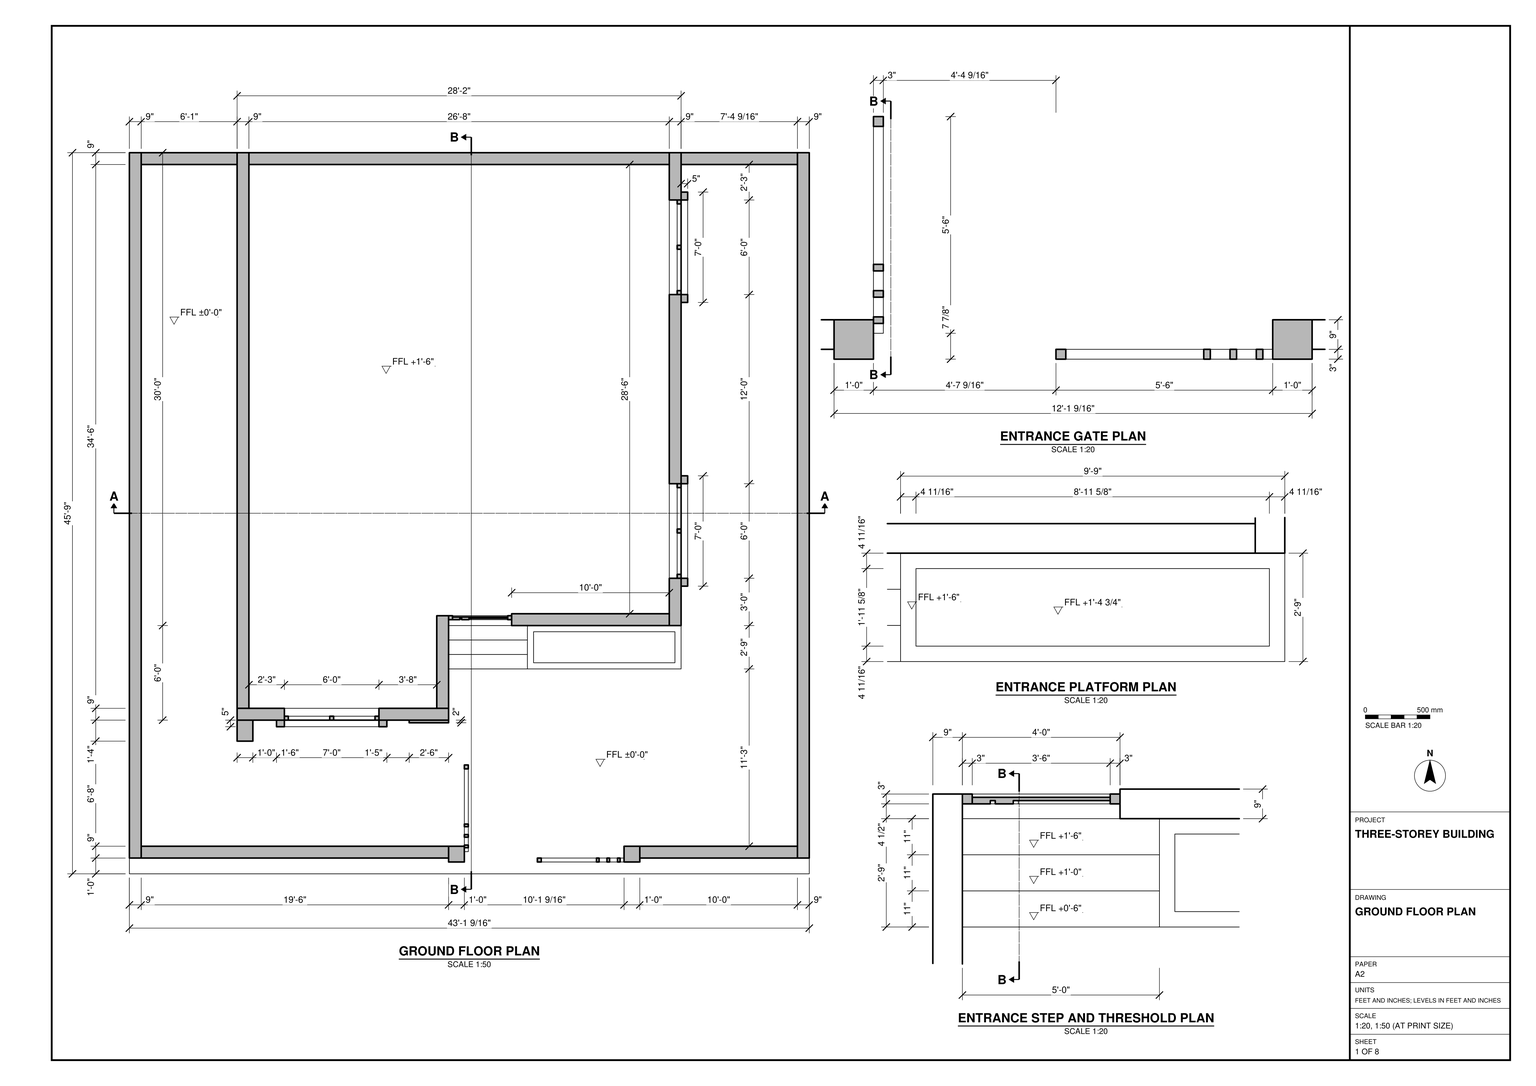
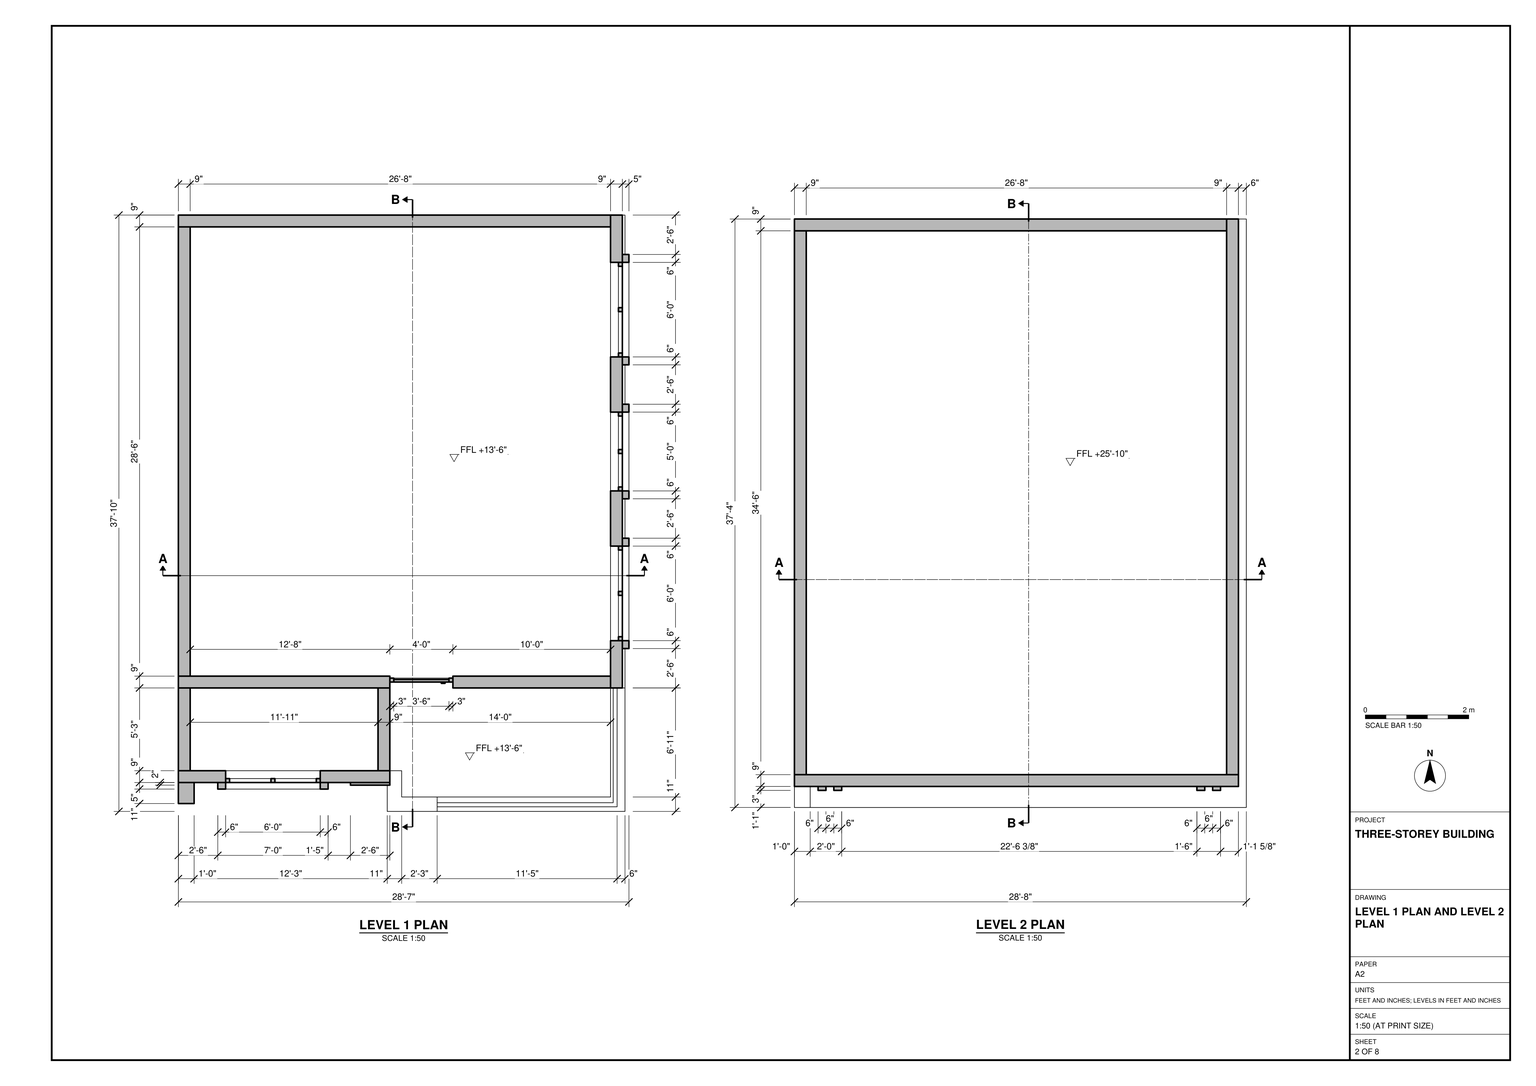
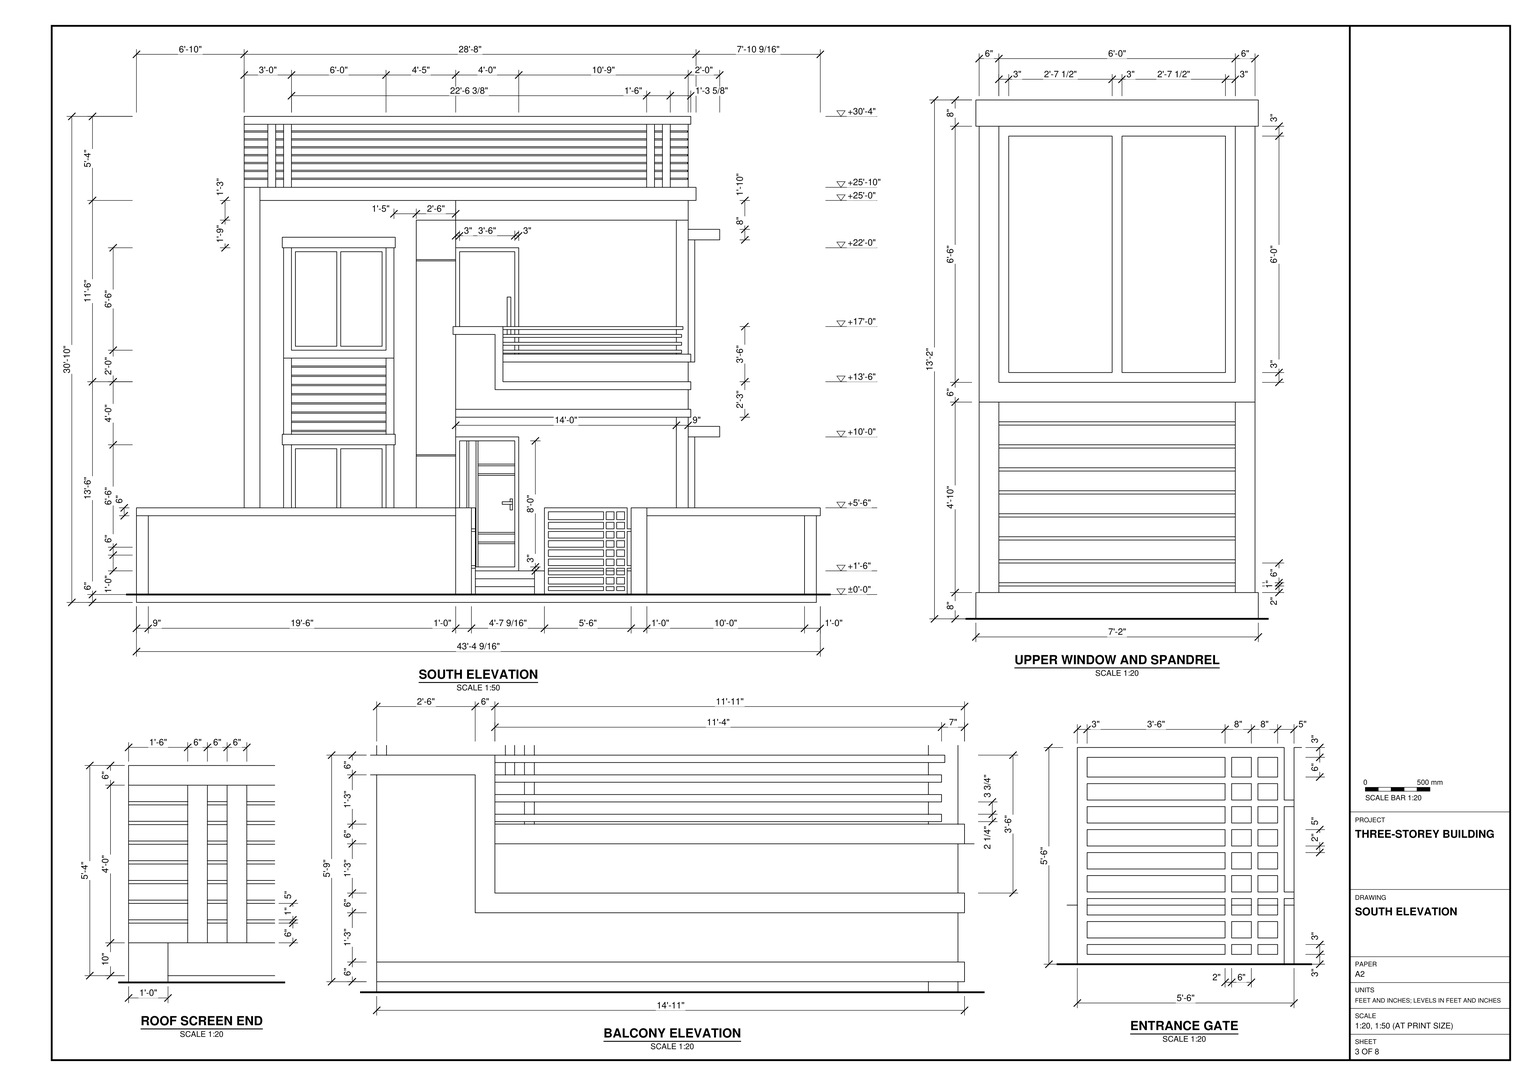
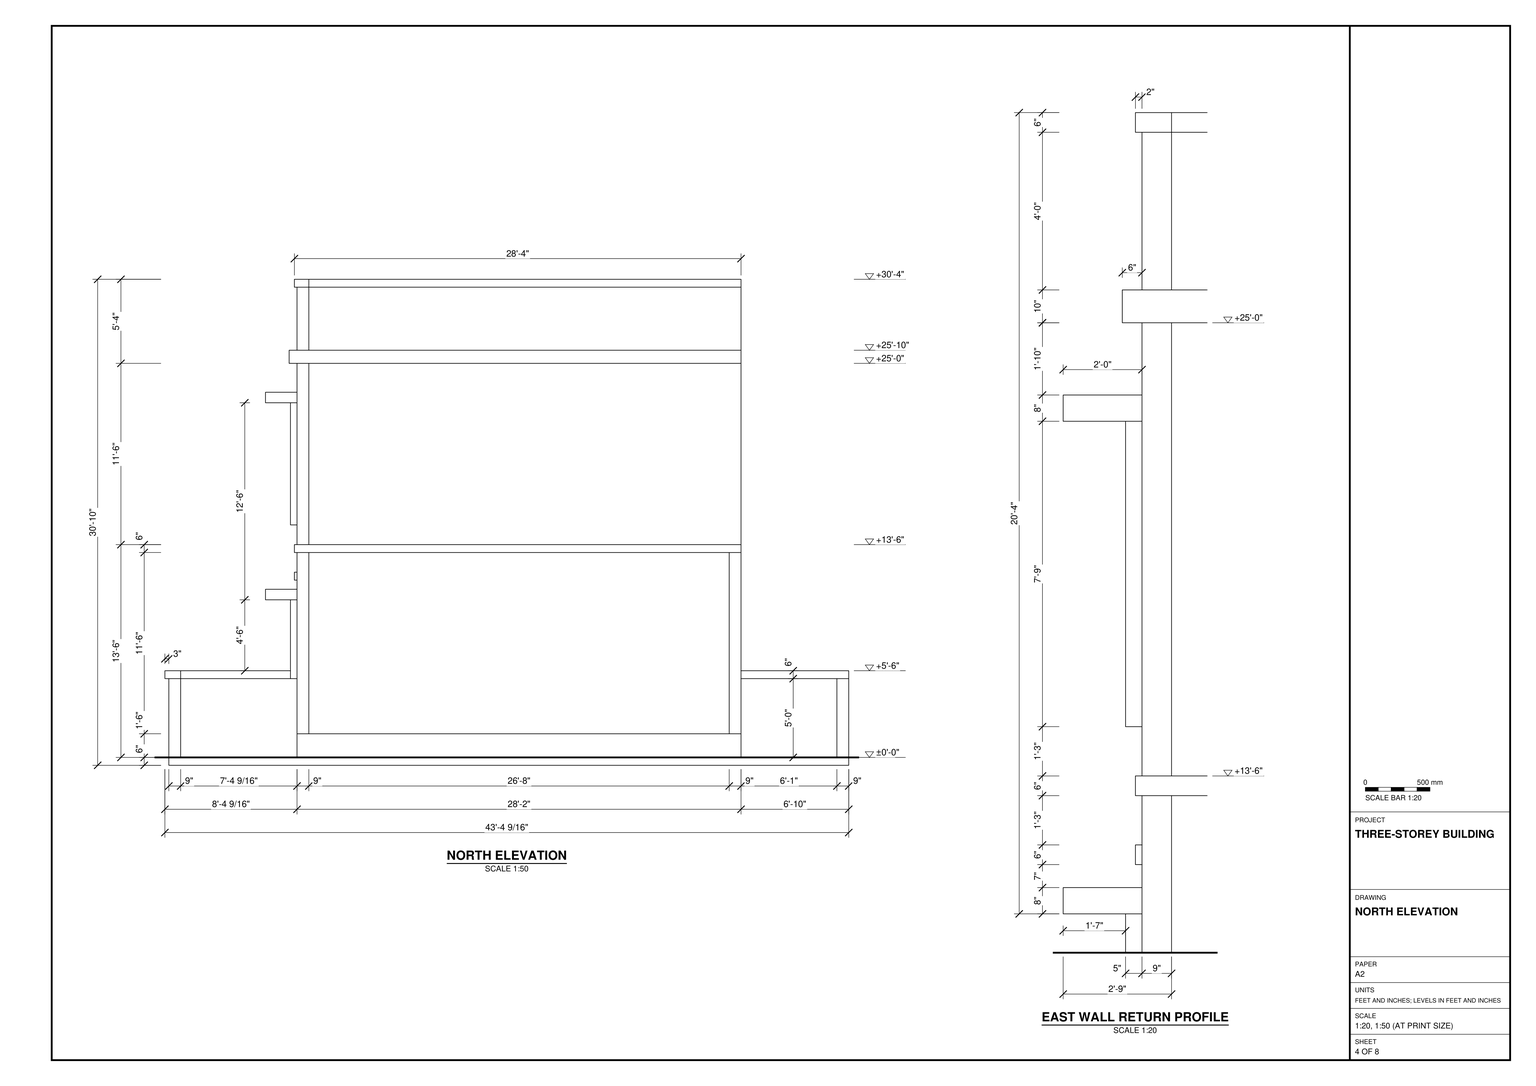
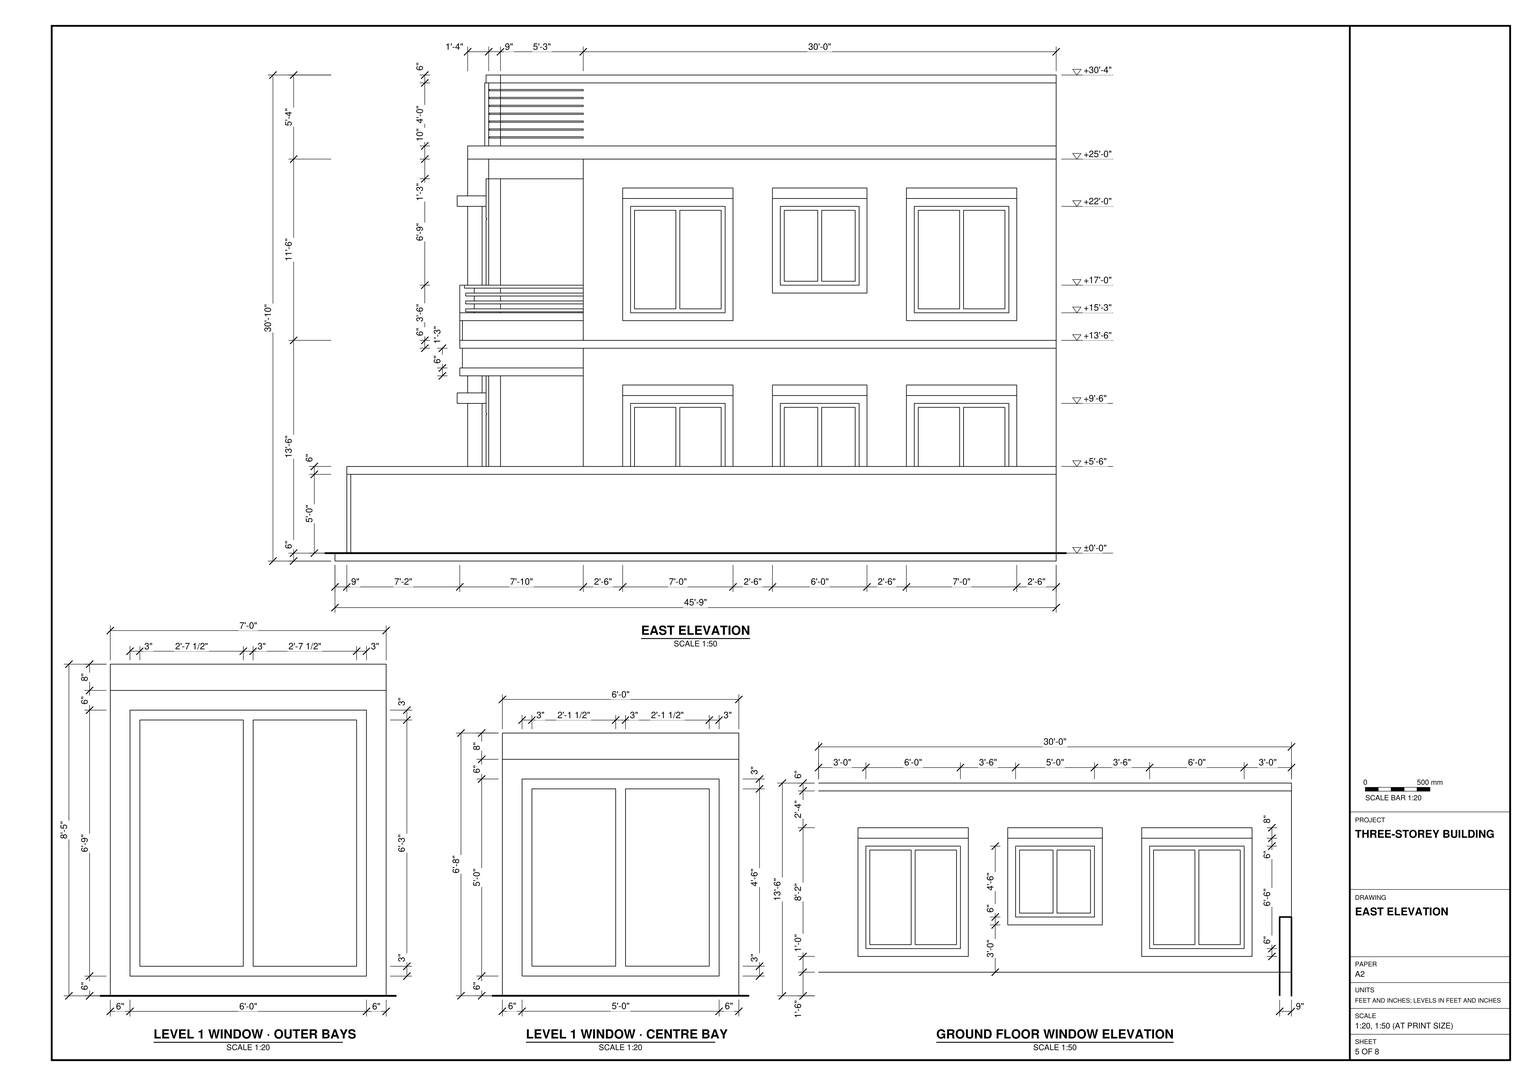
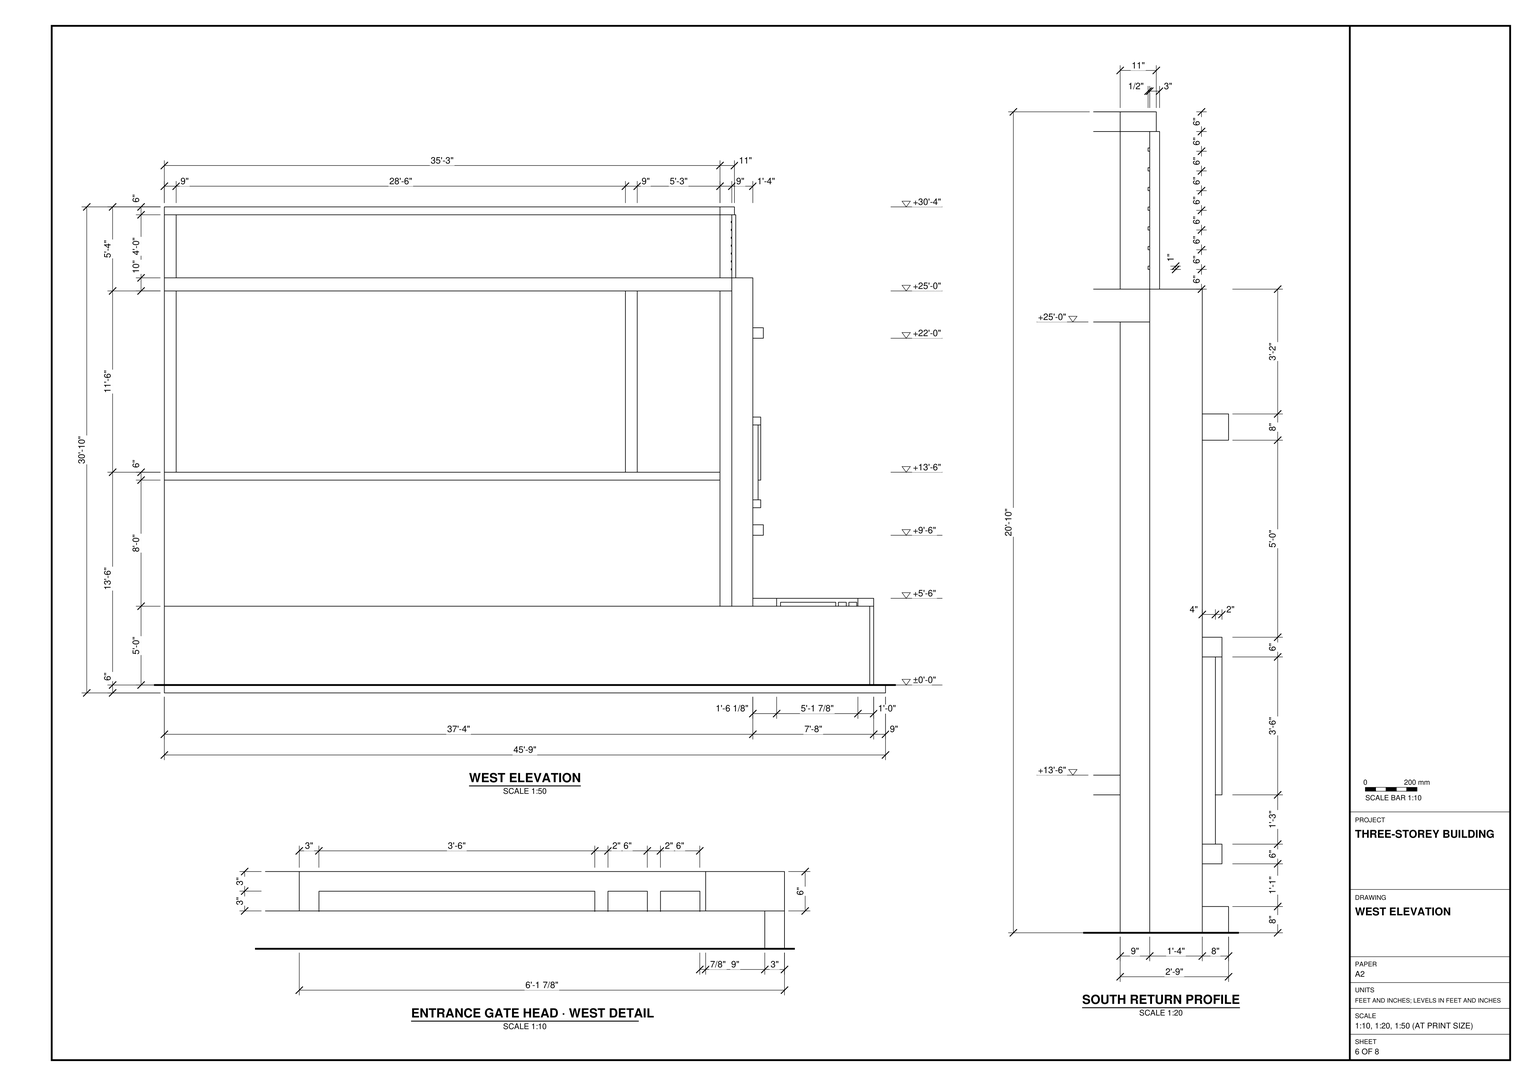
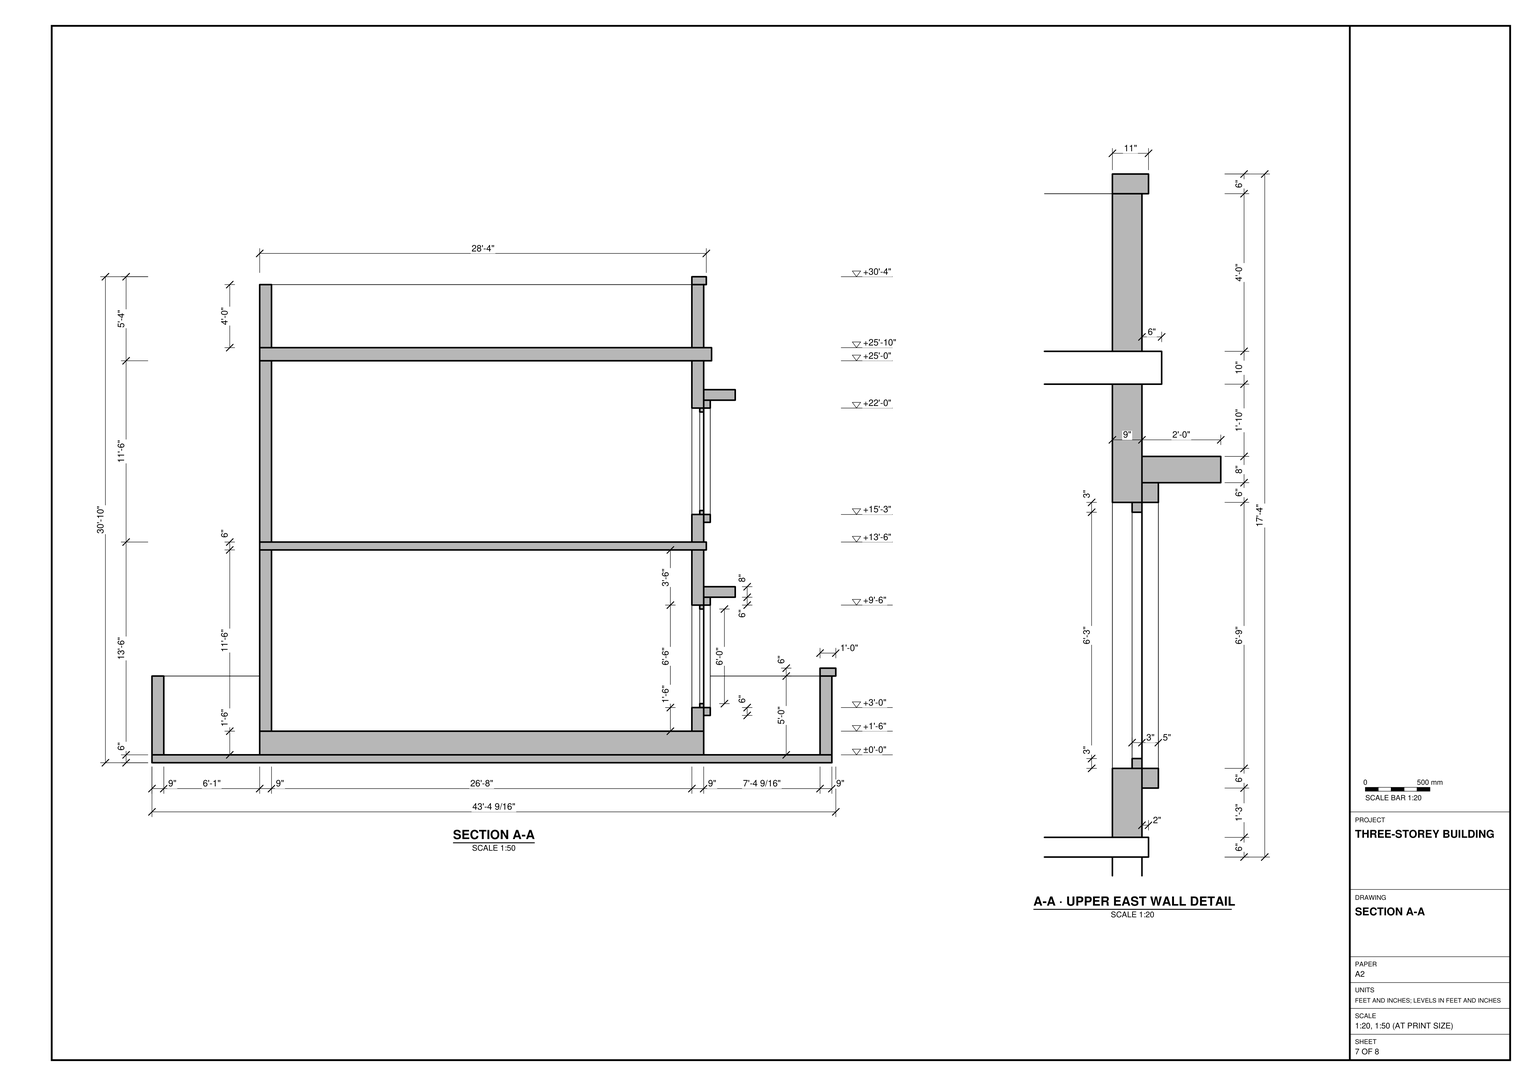
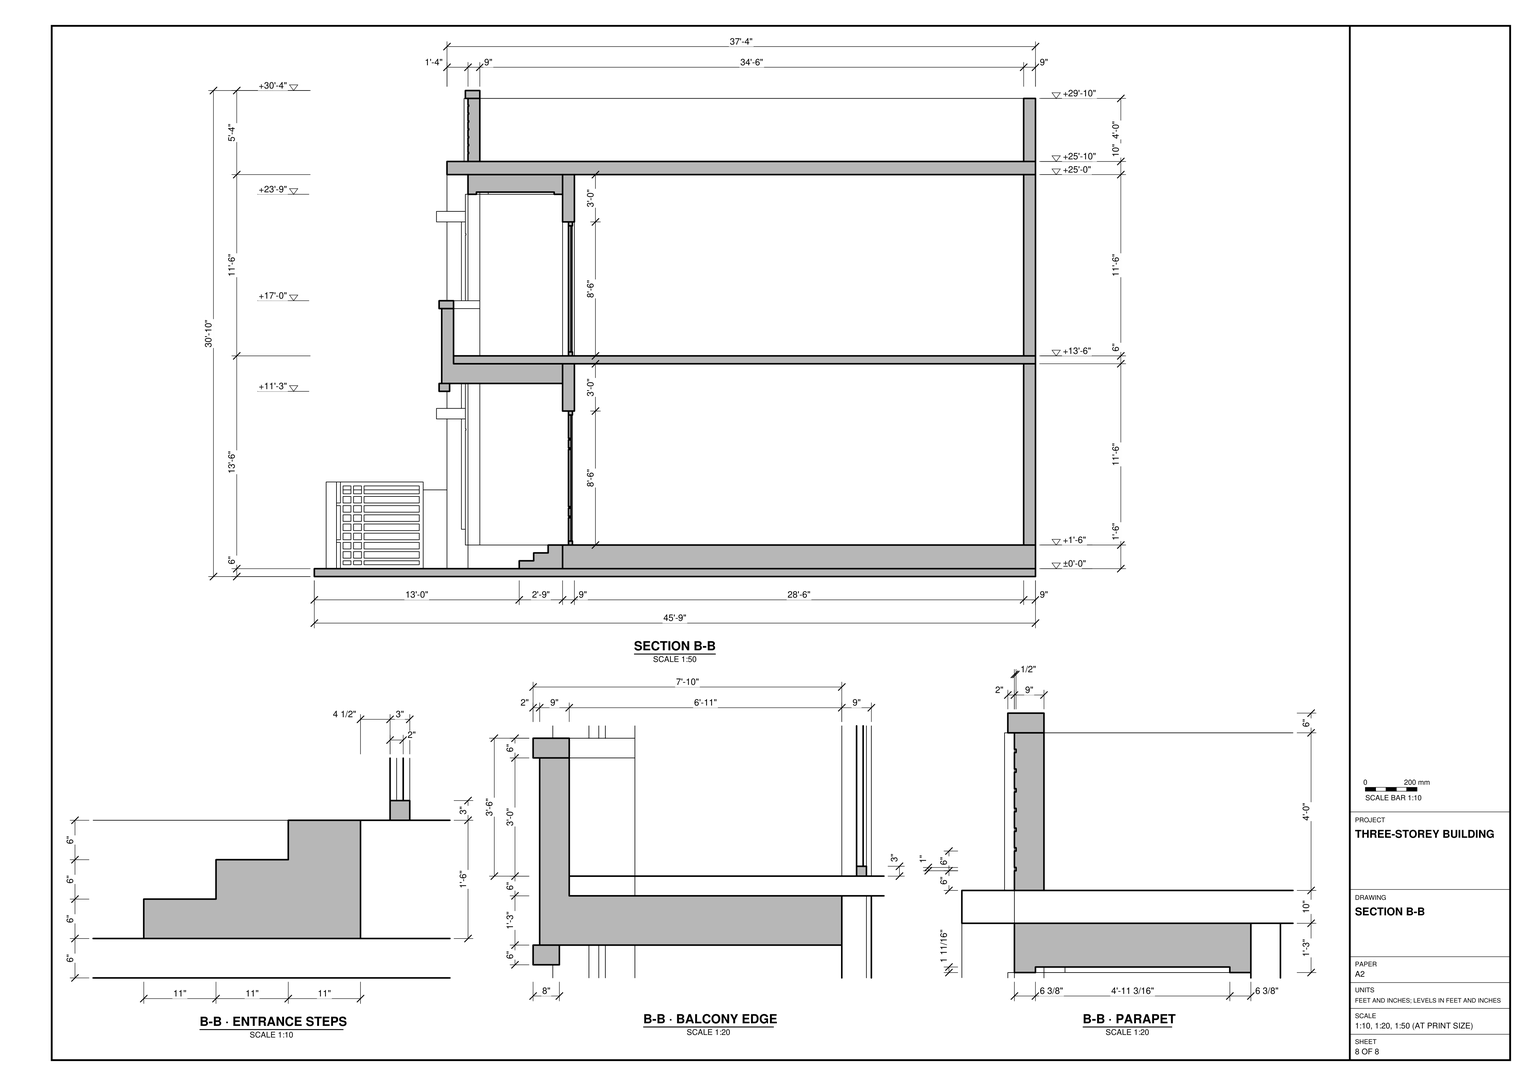
Build the three-storey building and its walled forecourt in SketchUp using task_files/diagram_01.pdf. Work in feet and inches. The overall model is 43'-4 9/16" across the south frontage, 45'-9" from front to back and 30'-10" from its lowest to its highest point. Use ±0'-0", +13'-6" and +25'-0" as the level references. Distinguish the forecourt at ±0'-0" from the raised ground-floor interior at +1'-6".

Lay out the boundary walls, gateposts and gate leaves from the ground-floor plan. Set the building back from the gate, with the projecting window bay to the left of the recessed entrance. Model the entrance steps, threshold and adjoining platform. Give the walls their drawn thicknesses, including the 9" main walls, and cut the door and window openings through them. Align the south windows vertically with the slatted spandrel between them. On the upper floor, model the door onto the front balcony, its solid lower face and its horizontal rails. Follow the plans for the east windows, floor slabs and flat roof, and use the elevation detail for the slats, uprights and cap of the roof screen.

Keep walls, slabs, roof elements and any furniture or joinery pieces in separate groups or components; use components for repeated parts. Decor and loose items, if included, may be any suitable library components. Save one SketchUp model as output_files/three_storey_building_with_gated_forecourt_and_balcony.skp.

# SketchUp Ruby script. Lengths in inches.
U = 1.inch
M = Sketchup.active_model
def pt(a) = Geom::Point3d.new(a.map { |v| v * U })
def face(e, loops, mat)
  f = e.add_face(loops[0].map { |a| pt(a) })
  loops[1..].each { |l| e.add_face(l.map { |a| pt(a) }).erase! }
  f.material = f.back_material = mat if mat
  f
end
# faces: each face lists its corners as indices into pts; further lists are holes
def faces(e, pts, list, mat = nil) = list.each { |f| face(e, (f[0].is_a?(Array) ? f : [f]).map { |l| l.map { |i| pts[i] } }, mat) }
# xy, xz, yz: faces in a plane at the given z, y or x. An outline is a flat list of corners, or four numbers for a rectangle; further outlines are holes
def ring(l) = l.size == 4 ? [[l[0], l[1]], [l[2], l[1]], [l[2], l[3]], [l[0], l[3]]] : l.each_slice(2).to_a
def flat(e, list, mat, &to3) = list.each { |f| face(e, (f[0].is_a?(Array) ? f : [f]).map { |l| ring(l).map { |u, v| to3.(u, v) } }, mat) }
def xy(e, z, list, mat = nil) = flat(e, list, mat) { |x, y| [x, y, z] }
def xz(e, y, list, mat = nil) = flat(e, list, mat) { |x, z| [x, y, z] }
def yz(e, x, list, mat = nil) = flat(e, list, mat) { |y, z| [x, y, z] }
def lines(e, pts, list) = list.each { |a, b| e.add_line(pt(pts[a]), pt(pts[b])) }
# prism: a flat outline (further loops are holes) pulled along v
def prism(e, loops, v, mat = nil)
  f = face(e, loops, mat); d = Geom::Vector3d.new(v.map { |x| x * U })
  f.pushpull(f.normal.samedirection?(d) ? d.length : -d.length)
end
def box(e, o, s, mat = nil) = prism(e, [[o, [o[0] + s[0], o[1], o[2]], [o[0] + s[0], o[1] + s[1], o[2]], [o[0], o[1] + s[1], o[2]]]], [0, 0, s[2]], mat)
def at(x, y, z, deg = 0) = Geom::Transformation.translation(pt([x, y, z])) * Geom::Transformation.rotation(ORIGIN, Z_AXIS, deg.degrees)
def axes(o, x, y, z) = Geom::Transformation.new([*x, 0, *y, 0, *z, 0, *pt(o).to_a, 1])
def part(name) = M.definitions.add(name)
# library, detail: a bought-in or finely detailed component or shape, given as its bounding box
def library(name, o, s) = part(name).tap { |d| box(d.entities, o, s) }
def detail(e, o, s) = box(e.add_group.entities, o, s)
def put(e, d, t, mat = nil) = e.add_instance(d, t).tap { |i| i.material = mat if mat }
def group(e, t, mat = nil) = e.add_group.tap { |g| g.transformation = t; g.material = mat if mat }.entities
root = M.entities
M.materials.add("[Aluminum]").color = [179, 179, 179]
M.materials.add("[Color C01]").color = [247, 234, 234]
M.materials.add("[Color C02]").color = [183, 146, 110]
M.materials.add("[Color M00]").color = [255, 255, 255]
M.materials.add("[Color M02]").color = [198, 198, 198]
M.materials.add("[Color M06]").color = [86, 86, 86]
M.materials.add("[Color M07]").color = [58, 58, 58]
M.materials.add("[Grass Dark Green]").color = [106, 157, 55]
M.materials.add("[Translucent Glass Gray]").color = [128, 128, 128]
M.materials["[Translucent Glass Gray]"].alpha = 0.5
M.materials.add("[Wood Veneer 01]").color = [120, 70, 37]
c1 = part("Group\#74")
box(c1.entities,[0,0,0],[6,3,48])
box(c1.entities,[12,0,0],[6,3,48])
c2 = part("Group\#93")
prism(c2.entities,[[[0,0,0],[63,0,0],[63,0,20],[66,0,20],[66,0,22],[63,0,22],[63,0,48],[66,0,48],[66,0,50],[63,0,50],[63,0,66],[0,0,66]],[[3,0,63],[45,0,63],[45,0,57],[3,0,57]],[[3,0,13],[45,0,13],[45,0,8],[3,0,8]],[[3,0,20],[45,0,20],[45,0,15],[3,0,15]],[[3,0,27],[45,0,27],[45,0,22],[3,0,22]],[[3,0,34],[45,0,34],[45,0,29],[3,0,29]],[[3,0,41],[45,0,41],[45,0,36],[3,0,36]],[[3,0,48],[45,0,48],[45,0,43],[3,0,43]],[[45,0,55],[45,0,50],[3,0,50],[3,0,55]],[[45,0,6],[45,0,3],[3,0,3],[3,0,6]],[[55,0,63],[61,0,63],[61,0,57],[55,0,57]],[[53,0,57],[47,0,57],[47,0,63],[53,0,63]],[[61,0,8],[55,0,8],[55,0,13],[61,0,13]],[[61,0,20],[61,0,15],[55,0,15],[55,0,20]],[[53,0,15],[47,0,15],[47,0,20],[53,0,20]],[[61,0,27],[61,0,22],[55,0,22],[55,0,27]],[[53,0,29],[47,0,29],[47,0,34],[53,0,34]],[[53,0,41],[53,0,36],[47,0,36],[47,0,41]],[[53,0,48],[53,0,43],[47,0,43],[47,0,48]],[[61,0,50],[55,0,50],[55,0,55],[61,0,55]],[[53,0,50],[47,0,50],[47,0,55],[53,0,55]],[[61,0,48],[61,0,43],[55,0,43],[55,0,48]],[[61,0,41],[61,0,36],[55,0,36],[55,0,41]],[[61,0,29],[55,0,29],[55,0,34],[61,0,34]],[[53,0,27],[53,0,22],[47,0,22],[47,0,27]],[[53,0,8],[47,0,8],[47,0,13],[53,0,13]],[[61,0,6],[61,0,3],[55,0,3],[55,0,6]],[[47,0,3],[47,0,6],[53,0,6],[53,0,3]]],[0,3,0])
p = [[66,3,22],[66,3,48],[66,3,0],[66,3,20],[66,3,50],[66,3,66]]
lines(c2.entities,p,[[0,1],[2,3],[4,5]])
p = [[94,112.99,306],[94,116.99,306]]
lines(root,p,[[0,1]])
g1 = group(root,at(142.63,241.1875,0))
box(g1,[-142.63,-241.1875,0],[517.57,548.99,6])
g2 = group(root,at(180,308.99,6),"[Color C01]")
prism(g2,[[[-98,240,0],[240,240,0],[240,-120,0],[63,-120,0],[63,-192,0],[-98,-192,0]]],[0,0,18])
g3 = group(root,at(411,308.99,24),"[Color C01]")
prism(g3,[[[0,240,0],[0,-120,0],[0,-120,138],[0,240,138]],[[0,132,96],[0,132,18],[0,204,18],[0,204,96]],[[0,-12,96],[0,-84,96],[0,-84,18],[0,-12,18]],[[0,90,96],[0,30,96],[0,30,42],[0,90,42]]],[9,0,0])
g4 = group(root,at(420,434.99,36),"[Color M06]")
prism(g4,[[[0,0,90],[0,84,90],[0,84,0],[0,0,0]],[[0,78,84],[0,6,84],[0,6,6],[0,78,6]]],[5,0,0])
g5 = group(root,at(417,440.99,42),"[Aluminum]")
prism(g5,[[[0,0,78],[0,72,78],[0,72,0],[0,0,0]],[[0,37.5,75],[0,37.5,3],[0,69,3],[0,69,75]],[[0,34.5,75],[0,3,75],[0,3,3],[0,34.5,3]]],[3,0,0])
g6 = group(root,at(420,478.49,45),"[Translucent Glass Gray]")
yz(g6,0,[[0,0,31.5,72]])
g7 = group(root,at(420,443.99,45),"[Translucent Glass Gray]")
yz(g7,0,[[0,0,31.5,72]])
g8 = group(root,at(420,332.99,60),"[Color M06]")
prism(g8,[[[0,0,0],[0,0,66],[0,72,66],[0,72,0]],[[0,66,60],[0,6,60],[0,6,6],[0,66,6]]],[5,0,0])
g9 = group(root,at(417,338.99,66),"[Aluminum]")
prism(g9,[[[0,60,0],[0,0,0],[0,0,54],[0,60,54]],[[0,28.5,3],[0,28.5,51],[0,3,51],[0,3,3]],[[0,31.5,3],[0,57,3],[0,57,51],[0,31.5,51]]],[3,0,0])
g10 = group(root,at(420,218.99,36),"[Color M06]")
prism(g10,[[[5,0,90],[5,0,0],[5,84,0],[5,84,90]],[[5,6,6],[5,6,84],[5,78,84],[5,78,6]]],[-5,0,0])
g11 = group(root,at(417,224.99,42),"[Aluminum]")
prism(g11,[[[3,0,0],[3,72,0],[3,72,78],[3,0,78]],[[3,37.5,3],[3,37.5,75],[3,69,75],[3,69,3]],[[3,3,75],[3,34.5,75],[3,34.5,3],[3,3,3]]],[-3,0,0])
g12 = group(root,at(420,262.49,45),"[Translucent Glass Gray]")
yz(g12,0,[[0,0,31.5,72]])
g13 = group(root,at(420,227.99,45),"[Translucent Glass Gray]")
yz(g13,0,[[0,0,31.5,72]])
g14 = group(root,at(420,370.49,69),"[Translucent Glass Gray]")
yz(g14,0,[[0,0,25.5,48]])
g15 = group(root,at(420,341.99,69),"[Translucent Glass Gray]")
yz(g15,0,[[0,0,25.5,48]])
g16 = group(root,at(420,218.99,126),"[Color M02]")
box(g16,[0,0,0],[24,84,8])
g17 = group(root,at(420,332.99,126),"[Color M02]")
box(g17,[0,0,0],[24,72,8])
g18 = group(root,at(420,434.99,126),"[Color M02]")
box(g18,[0,0,0],[24,84,8])
g19 = group(root,at(300,188.99,24),"[Color C01]")
prism(g19,[[[111,9,0],[-9,9,0],[-9,9,102],[-57,9,102],[-57,9,138],[111,9,138]]],[0,-9,0])
g20 = group(root,at(243,193.49,24),"[Wood Veneer 01]")
prism(g20,[[[0,3,0],[0,3,102],[48,3,102],[48,3,0]],[[45,3,99],[3,3,99],[3,3,3],[45,3,3]]],[0,-3,0])
g21 = group(root,at(246,193.49,27),"[Wood Veneer 01]")
xy(g21,0,[[0,0,0,2,42,2,42,0,14,0,14,1,12.5,1,12.5,0,7,0,7,1,5.5,1,5.5,0]])
xy(g21,17.7,[[14,0,42,1]])
xy(g21,19,[[14,0,42,1]])
xy(g21,25,[[14,0,42,1]])
xy(g21,26.3,[[14,0,42,1]])
xy(g21,69.7,[[14,0,42,1]])
xy(g21,71,[[14,0,42,1]])
xy(g21,77,[[14,0,42,1]])
xy(g21,78.3,[[14,0,42,1]])
xy(g21,96,[[0,0,5.5,0,5.5,1,7,1,7,0,12.5,0,12.5,1,14,1,14,0,42,0,42,2,0,2]])
xz(g21,0,[[0,0,5.5,96],[7,0,12.5,96],[14,0,42,17.7],[14,19,42,25],[14,26.3,42,69.7],
  [14,71,42,77],[14,78.3,42,96]])
xz(g21,1,[[5.5,0,7,96],[12.5,0,14,96],[14,17.7,42,19],[14,25,42,26.3],[14,69.7,42,71],
  [14,77,42,78.3]],"[Color M00]")
xz(g21,2,[[0,0,42,96]])
yz(g21,0,[[0,0,2,96]])
yz(g21,5.5,[[0,0,1,96]])
yz(g21,7,[[0,0,1,96]])
yz(g21,12.5,[[0,0,1,96]])
yz(g21,14,[[0,0,1,17.7],[0,19,1,25],[0,26.3,1,69.7],[0,71,1,77],[0,78.3,1,96]])
yz(g21,42,[[0,0,2,0,2,96,0,96,0,78.3,1,78.3,1,77,0,77,0,71,1,71,1,69.7,0,69.7,0,26.3,1,26.3,1,25,0,25,0,19,1,19,1,17.7,0,17.7]])
g22 = group(root,at(284.43,191.49,67.4375),"[Aluminum]")
box(g22,[0,0,2.9375],[1.8125,2,8.4375])
g23 = group(root,at(278.43,190.49,74.65),"[Aluminum]")
box(g23,[0,0,0],[7.8125,1,1.97])
g24 = group(root,at(234,116.99,24),"[Color C02]")
box(g24,[0,9,0],[9,70.5,138])
g25 = group(root,at(63,116.99,24),"[Color C01]")
xy(g25,0,[[19,0,180,9]])
xy(g25,18,[[55,0,127,9]])
xy(g25,96,[[55,0,127,9]])
xy(g25,168,[[55,0,127,9]])
xy(g25,246,[[55,0,127,9]])
xy(g25,282,[[19,0,180,9]])
xz(g25,0,[[[19,0,180,282],[55,18,127,96],[55,168,127,246]]])
xz(g25,9,[[[19,0,180,282],[55,18,127,96],[55,168,127,246]]])
yz(g25,19,[[0,0,9,282]])
yz(g25,55,[[0,18,9,96],[0,168,9,246]])
yz(g25,127,[[0,18,9,96],[0,168,9,246]])
yz(g25,180,[[0,0,9,282]],"[Color C02]")
g26 = group(root,at(112,111.99,36),"[Color M06]")
xy(g26,0,[[0,0,84,5]])
xy(g26,6,[[6,0,78,5]])
xy(g26,150,[[0,0,6,5],[78,0,84,5]])
xz(g26,0,[[0,0,84,0,84,150,78,150,78,6,6,6,6,150,0,150]])
xz(g26,5,[[0,0,0,150,6,150,6,6,78,6,78,150,84,150,84,0]])
yz(g26,0,[[0,0,5,150]])
yz(g26,6,[[0,6,5,150]])
yz(g26,78,[[0,6,5,150]])
yz(g26,84,[[0,0,5,150]])
p = [[78,5,84],[6,5,84]]
lines(g26,p,[[0,1]])
g27 = group(root,at(118,116.99,42),"[Aluminum]")
prism(g27,[[[72,3,0],[0,3,0],[0,3,78],[72,3,78]],[[34.5,3,3],[34.5,3,75],[3,3,75],[3,3,3]],[[69,3,75],[37.5,3,75],[37.5,3,3],[69,3,3]]],[0,-3,0])
g28 = group(root,at(121,116.99,45),"[Translucent Glass Gray]")
xz(g28,0,[[0,0,31.5,72]])
g29 = group(root,at(155.5,116.99,45),"[Translucent Glass Gray]")
xz(g29,0,[[0,0,31.5,72]])
g30 = group(root,at(213,114.99,24),"[Color C02]")
prism(g30,[[[30,2,0],[30,2,267],[30,0,267],[30,0,237],[30,0.5,237],[30,0.5,236],[30,0,236],[30,0,88.44],[30,0.5,88.44],[30,0.5,87.44],[30,0,87.44],[30,0,0]]],[-30,0,0])
g31 = group(root,at(63,125.99,162),"[Color M06]")
xy(g31,0,[[210,-31,210,-20,189,-20,189,0,19,0,19,423,359,423,359,-31]])
xy(g31,6,[[216,-31,359,-31,359,423,19,423,19,0,189,0,189,-20,216,-20]])
xy(g31,42,[[178,-31,178,0,189,0,189,-20,210,-20,210,-31]])
xy(g31,48,[[178,-31,216,-31,216,-20,189,-20,189,0,178,0]])
xz(g31,-31,[[210,0,359,0,359,6,216,6,216,48,178,48,178,42,210,42]])
xz(g31,-20,[[189,0,210,6],[210,6,210,42,189,42,189,48,216,48,216,6]])
xz(g31,0,[[19,0,189,6],[178,42,189,48]])
xz(g31,423,[[19,0,359,6]])
yz(g31,19,[[0,0,423,6]])
yz(g31,178,[[-31,42,0,48]])
yz(g31,189,[[-20,0,0,6],[-20,42,0,48]])
yz(g31,210,[[-31,0,-20,42]])
yz(g31,216,[[-31,6,-20,48]])
yz(g31,359,[[-31,0,423,6]])
g32 = group(root,at(252,96.99,147),"[Color C02]")
xy(g32,0,[[-9,0,168,92]])
xy(g32,15,[[21,0,168,0,168,92,-9,92,-9,9,21,9]])
xy(g32,57,[[-9,0,21,9]])
xz(g32,0,[[-9,0,168,0,168,15,21,15,21,57,-9,57]])
xz(g32,9,[[-9,15,21,57]])
xz(g32,92,[[-9,0,168,15]])
yz(g32,-9,[[0,0,0,57,9,57,9,15,92,15,92,0]])
yz(g32,21,[[0,15,9,57]])
yz(g32,168,[[0,0,92,15]])
g33 = group(root,at(252,94.99,141),"[Color M06]")
prism(g33,[[[170,94,0],[170,0,0],[-9,0,0],[-9,8,0],[162,8,0],[162,94,0]]],[0,0,6])
g34 = group(root,at(279,96.99,168),"[Color C02]")
prism(g34,[[[0,0,0],[0,9,0],[132,9,0],[132,92,0],[141,92,0],[141,0,0]]],[0,0,15])
g35 = group(root,at(279,94.99,183),"[Color M06]")
prism(g35,[[[0,0,0],[0,11,0],[132,11,0],[132,94,0],[143,94,0],[143,0,0]]],[0,0,6])
g36 = group(root,at(411,188.99,168),"[Color C01]")
prism(g36,[[[0,360,0],[0,0,0],[0,0,138],[0,360,138]],[[0,108,102],[0,36,102],[0,36,21],[0,108,21]],[[0,324,102],[0,252,102],[0,252,21],[0,324,21]],[[0,210,102],[0,150,102],[0,150,42],[0,210,42]]],[9,0,0])
g37 = group(root,at(82,188.99,168),"[Color C01]")
prism(g37,[[[329,9,0],[209,9,0],[209,9,102],[161,9,102],[161,9,0],[0,9,0],[0,9,138],[329,9,138]]],[0,-9,0])
g38 = group(root,at(420,434.99,183),"[Color M06]")
prism(g38,[[[0,84,93],[0,84,0],[0,0,0],[0,0,93]],[[0,78,87],[0,6,87],[0,6,6],[0,78,6]]],[5,0,0])
g39 = group(root,at(420,332.99,204),"[Color M06]")
prism(g39,[[[0,0,72],[0,72,72],[0,72,0],[0,0,0]],[[0,66,66],[0,6,66],[0,6,6],[0,66,6]]],[5,0,0])
g40 = group(root,at(420,218.99,183),"[Color M06]")
prism(g40,[[[0,0,93],[0,84,93],[0,84,0],[0,0,0]],[[0,78,87],[0,6,87],[0,6,6],[0,78,6]]],[5,0,0])
g41 = group(root,at(417,224.99,189),"[Aluminum]")
prism(g41,[[[0,0,81],[0,72,81],[0,72,0],[0,0,0]],[[0,37.5,78],[0,37.5,3],[0,69,3],[0,69,78]],[[0,34.5,78],[0,3,78],[0,3,3],[0,34.5,3]]],[3,0,0])
g42 = group(root,at(420,262.49,192),"[Translucent Glass Gray]")
yz(g42,0,[[0,0,31.5,75]])
g43 = group(root,at(420,227.99,192),"[Translucent Glass Gray]")
yz(g43,0,[[0,0,31.5,75]])
g44 = group(root,at(417,338.99,210),"[Aluminum]")
prism(g44,[[[0,0,60],[0,60,60],[0,60,0],[0,0,0]],[[0,31.5,57],[0,31.5,3],[0,57,3],[0,57,57]],[[0,28.5,57],[0,3,57],[0,3,3],[0,28.5,3]]],[3,0,0])
g45 = group(root,at(420,370.49,213),"[Translucent Glass Gray]")
yz(g45,0,[[0,0,25.5,54]])
g46 = group(root,at(420,341.99,213),"[Translucent Glass Gray]")
yz(g46,0,[[0,0,25.5,54]])
g47 = group(root,at(417,440.99,189),"[Aluminum]")
prism(g47,[[[0,0,81],[0,72,81],[0,72,0],[0,0,0]],[[0,37.5,3],[0,69,3],[0,69,78],[0,37.5,78]],[[0,34.5,3],[0,34.5,78],[0,3,78],[0,3,3]]],[3,0,0])
g48 = group(root,at(420,478.49,192),"[Translucent Glass Gray]")
yz(g48,0,[[0,0,31.5,75]])
g49 = group(root,at(420,443.99,192),"[Translucent Glass Gray]")
yz(g49,0,[[0,0,31.5,75]])
g50 = group(root,at(243,193.49,168),"[Wood Veneer 01]")
prism(g50,[[[0,3,0],[0,3,102],[48,3,102],[48,3,0]],[[45,3,3],[45,3,99],[3,3,99],[3,3,3]]],[0,-3,0])
g51 = group(root,at(246,193.49,171),"[Wood Veneer 01]")
box(g51,[0,0,0],[42,2,96])
g52 = group(root,at(420,218.99,276),"[Color M02]")
box(g52,[0,0,0],[24,84,8])
g53 = group(root,at(420,332.99,276),"[Color M02]")
box(g53,[0,0,0],[24,72,8])
g54 = group(root,at(420,434.99,276),"[Color M02]")
box(g54,[0,0,0],[24,84,8])
g55 = group(root,at(282.19,192.49,203.23),"[Aluminum]")
box(g55,[0,0,0],[2.8125,1,29.25])
g56 = group(root,at(112,111.99,186),"[Color M06]")
prism(g56,[[[84,0,84],[78,0,84],[78,0,6],[6,0,6],[6,0,84],[0,0,84],[0,0,0],[84,0,0]]],[0,5,0])
p = [[78,5,84],[6,5,84]]
lines(g56,p,[[0,1]])
g57 = group(root,at(118,116.99,192),"[Aluminum]")
prism(g57,[[[72,3,0],[0,3,0],[0,3,78],[72,3,78]],[[37.5,3,75],[37.5,3,3],[69,3,3],[69,3,75]],[[3,3,3],[34.5,3,3],[34.5,3,75],[3,3,75]]],[0,-3,0])
g58 = group(root,at(155.5,116.99,195),"[Translucent Glass Gray]")
xz(g58,0,[[0,0,31.5,72]])
g59 = group(root,at(121,116.99,195),"[Translucent Glass Gray]")
xz(g59,0,[[0,0,31.5,72]])
g60 = group(root,at(112,92.99,120),"[Color M02]")
box(g60,[-1,0,0],[86,24,8])
g61 = group(root,at(112,92.99,270),"[Color M02]")
box(g61,[-1,0,0],[86,24,8])
g62 = group(root,at(118,113.99,128),"[Color C02]")
prism(g62,[[[72,3,0],[72,3,58],[72,0,58],[72,0,52],[72,0.5,52],[72,0.5,51],[72,0,51],[72,0,45],[72,0.5,45],[72,0.5,44],[72,0,44],[72,0,38],[72,0.5,38],[72,0.5,37],[72,0,37],[72,0,31],[72,0.5,31],[72,0.5,30],[72,0,30],[72,0,24],[72,0.5,24],[72,0.5,23],[72,0,23],[72,0,17],[72,0.5,17],[72,0.5,16],[72,0,16],[72,0,10],[72,0.5,10],[72,0.5,9],[72,0,9],[72,0,3],[72,0.5,3],[72,0.5,2],[72,0,2],[72,0,0]]],[-72,0,0])
g63 = group(root,at(82,188.99,306),"[Color M06]")
prism(g63,[[[0,360,0],[344,360,0],[344,-88,0],[12,-88,0],[12,-72,0],[0,-72,0]]],[0,0,10])
g64 = group(root,at(243,96.99,291),"[Color C01]")
xy(g64,0,[[0,20,0,26.4,170.6,26.4,170.6,85.6,-145.6,85.6,-145.6,35.4,0,35.4,0,29,-152,29,-152,92,177,92,177,20]])
xy(g64,1.6875,[[0,26.4,0,35.4,-145.6,35.4,-145.6,85.6,170.6,85.6,170.6,26.4]],"[Color C02]")
xy(g64,15,[[0,20,177,20,177,92,-152,92,-152,29,0,29]])
xz(g64,20,[[0,0,177,15]])
xz(g64,26.4,[[0,0,170.6,1.6875]])
xz(g64,29,[[-152,0,0,15]])
xz(g64,35.4,[[-145.6,0,0,1.6875]])
xz(g64,85.6,[[-145.6,0,170.6,1.6875]])
xz(g64,92,[[-152,0,177,15]])
yz(g64,-152,[[29,0,92,15]])
yz(g64,-145.6,[[35.4,0,85.6,1.6875]])
yz(g64,0,[[20,0,20,15,29,15,29,1.6875,26.4,1.6875,26.4,0],[26.4,0,29,1.6875],[29,0,35.4,1.6875]])
yz(g64,170.6,[[26.4,0,85.6,1.6875]])
yz(g64,177,[[20,0,92,15]])
g65 = group(root,at(82,125.99,168))
box(g65,[0,0,0],[9,63,138])
g66 = group(root,at(234,105.99,162),"[Color C02]")
xy(g66,0,[[9,0,18,20]])
xy(g66,6,[[0,20,9,83]])
xy(g66,42,[[9,0,18,20]])
xy(g66,129,[[0,20,9,83]])
xz(g66,0,[[9,0,18,42]])
xz(g66,20,[[9,0,18,42],[0,6,9,129]])
xz(g66,83,[[0,6,9,129]])
yz(g66,0,[[20,6,83,129]])
yz(g66,9,[[0,0,20,42],[20,6,83,129]])
yz(g66,18,[[0,0,20,42]])
p = [[9,9,48],[9,20,48],[7,9,48]]
lines(g66,p,[[0,1],[2,0]])
g67 = group(root,at(82,100.99,24),"[Color M06]")
box(g67,[0,0,-18],[12,16,310])
g68 = group(root,at(82,116.99,316),"[Color C01]")
xy(g68,0,[[0,0,338,9]])
xy(g68,6,[[0,0,338,0.5],[337.5,0.5,338,9]])
xy(g68,7,[[0,0,338,0.5],[337.5,0.5,338,9]])
xy(g68,12,[[0,0,338,0.5],[337.5,0.5,338,9]])
xy(g68,13,[[0,0,338,0.5],[337.5,0.5,338,9]])
xy(g68,18,[[0,0,338,0.5],[337.5,0.5,338,9]])
xy(g68,19,[[0,0,338,0.5],[337.5,0.5,338,9]])
xy(g68,24,[[0,0,338,0.5],[337.5,0.5,338,9]])
xy(g68,25,[[0,0,338,0.5],[337.5,0.5,338,9]])
xy(g68,30,[[0,0,338,0.5],[337.5,0.5,338,9]])
xy(g68,31,[[0,0,338,0.5],[337.5,0.5,338,9]])
xy(g68,36,[[0,0,338,0.5],[337.5,0.5,338,9]])
xy(g68,37,[[0,0,338,0.5],[337.5,0.5,338,9]])
xy(g68,42,[[0,0,338,0.5],[337.5,0.5,338,9]])
xy(g68,43,[[0,0,338,0.5],[337.5,0.5,338,9]])
xy(g68,48,[[0,0,338,9]])
xz(g68,0,[[0,0,338,6],[0,7,338,12],[0,13,338,18],[0,19,338,24],[0,25,338,30],
  [0,31,338,36],[0,37,338,42],[0,43,338,48]])
xz(g68,0.5,[[0,6,337.5,7],[0,12,337.5,13],[0,18,337.5,19],[0,24,337.5,25],[0,30,337.5,31],
  [0,36,337.5,37],[0,42,337.5,43]])
xz(g68,9,[[0,0,0,48,338,48,338,43,337.5,43,337.5,42,338,42,338,37,337.5,37,337.5,36,338,36,338,31,337.5,31,337.5,30,338,30,338,25,337.5,25,337.5,24,338,24,338,19,337.5,19,337.5,18,338,18,338,13,337.5,13,337.5,12,338,12,338,7,337.5,7,337.5,6,338,6,338,0]])
yz(g68,0,[[0,0,0,6,0.5,6,0.5,7,0,7,0,12,0.5,12,0.5,13,0,13,0,18,0.5,18,0.5,19,0,19,0,24,0.5,24,0.5,25,0,25,0,30,0.5,30,0.5,31,0,31,0,36,0.5,36,0.5,37,0,37,0,42,0.5,42,0.5,43,0,43,0,48,9,48,9,0]])
yz(g68,337.5,[[0.5,6,9,7],[0.5,12,9,13],[0.5,18,9,19],[0.5,24,9,25],[0.5,30,9,31],
  [0.5,36,9,37],[0.5,42,9,43]])
yz(g68,338,[[0,0,9,6],[0,7,9,12],[0,13,9,18],[0,19,9,24],[0,25,9,30],
  [0,31,9,36],[0,37,9,42],[0,43,9,48]])
g69 = group(root,at(411,125.99,316),"[Color C01]")
xy(g69,0,[[0,0,9,423]])
xy(g69,6,[[8.5,0,9,63]])
xy(g69,7,[[8.5,0,9,63]])
xy(g69,12,[[8.5,0,9,63]])
xy(g69,13,[[8.5,0,9,63]])
xy(g69,18,[[8.5,0,9,63]])
xy(g69,19,[[8.5,0,9,63]])
xy(g69,24,[[8.5,0,9,63]])
xy(g69,25,[[8.5,0,9,63]])
xy(g69,30,[[8.5,0,9,63]])
xy(g69,31,[[8.5,0,9,63]])
xy(g69,36,[[8.5,0,9,63]])
xy(g69,37,[[8.5,0,9,63]])
xy(g69,42,[[8.5,0,9,63]])
xy(g69,43,[[8.5,0,9,63]])
xy(g69,48,[[0,0,9,423]])
xz(g69,0,[[0,0,9,0,9,6,8.5,6,8.5,7,9,7,9,12,8.5,12,8.5,13,9,13,9,18,8.5,18,8.5,19,9,19,9,24,8.5,24,8.5,25,9,25,9,30,8.5,30,8.5,31,9,31,9,36,8.5,36,8.5,37,9,37,9,42,8.5,42,8.5,43,9,43,9,48,0,48]])
xz(g69,63,[[8.5,6,9,7],[8.5,12,9,13],[8.5,18,9,19],[8.5,24,9,25],[8.5,30,9,31],
  [8.5,36,9,37],[8.5,42,9,43]])
xz(g69,423,[[0,0,9,48]])
yz(g69,0,[[0,0,423,48]])
yz(g69,8.5,[[0,6,63,7],[0,12,63,13],[0,18,63,19],[0,24,63,25],[0,30,63,31],
  [0,36,63,37],[0,42,63,43]])
yz(g69,9,[[0,0,423,0,423,48,0,48,0,43,63,43,63,42,0,42,0,37,63,37,63,36,0,36,0,31,63,31,63,30,0,30,0,25,63,25,63,24,0,24,0,19,63,19,63,18,0,18,0,13,63,13,63,12,0,12,0,7,63,7,63,6,0,6]])
g70 = group(root,at(82,539.99,316))
box(g70,[0,0,0],[329,9,48])
g71 = group(root,at(82,125.99,316))
box(g71,[0,0,0],[9,414,48])
g72 = group(root,at(82,114.99,364),"[Color M06]")
box(g72,[0,0,0],[340,11,6])
g73 = group(root,at(411,125.99,364),"[Color M06]")
box(g73,[0,0,0],[11,423,6])
put(root,c1,at(100,113.99,316),"[Color M06]")
put(root,c1,at(388.375,113.99,316),"[Color M06]")
g74 = group(root,at(279,98.5,207.75),"[Color M07]")
prism(g74,[[[0,0,0],[0,3.125,0],[134,3.125,0],[134,90.49,0],[137,90.49,0],[137,0,0]]],[0,0,2.25])
g75 = group(root,at(279,98.5,201.75),"[Color M07]")
prism(g75,[[[0,1,0],[0,3.125,0],[134,3.125,0],[134,90.49,0],[136,90.49,0],[136,1,0]]],[0,0,2.25])
g76 = group(root,at(279,98.5,195.75),"[Color M07]")
prism(g76,[[[0,1,0],[0,3.125,0],[134,3.125,0],[134,90.49,0],[136,90.49,0],[136,1,0]]],[0,0,2.25])
g77 = group(root,at(279,98.5,189.75),"[Color M07]")
prism(g77,[[[0,1,0],[0,3.125,0],[134,3.125,0],[134,90.49,0],[136,90.49,0],[136,1,0]]],[0,0,2.25])
g78 = group(root,at(82,125.99,24))
box(g78,[0,0,0],[9,423,138])
g79 = group(root,at(91,539.99,24))
box(g79,[0,0,0],[320,9,138])
g80 = group(root,at(82,539.99,168))
box(g80,[0,0,0],[329,9,138])
g81 = group(root,at(82,197.99,168))
box(g81,[0,0,0],[9,342,138])
g82 = group(root,at(243,155.99,6),"[Color C01]")
xy(g82,0,[[0,0,60,33],[60,0,177,33]])
xy(g82,6,[[0,0,60,11]])
xy(g82,12,[[0,11,60,22]])
xy(g82,16.75,[[64.6875,4.6875,172.3125,28.3125]],"[Grass Dark Green]")
xy(g82,18,[[[60,0,177,33],[64.6875,4.6875,172.3125,28.3125]],[0,22,60,33]])
xz(g82,0,[[0,0,60,6],[60,0,177,18]])
xz(g82,4.6875,[[64.6875,16.75,172.3125,18]])
xz(g82,11,[[0,6,60,12]])
xz(g82,22,[[0,12,60,18]])
xz(g82,28.3125,[[64.6875,16.75,172.3125,18]])
xz(g82,33,[[0,0,60,18],[60,0,177,18]])
yz(g82,0,[[0,0,0,6,11,6,11,12,22,12,22,18,33,18,33,0]])
yz(g82,60,[[0,0,0,6,11,6,11,12,22,12,22,18,33,18,33,0],[0,6,0,18,22,18,22,12,11,12,11,6]])
yz(g82,64.6875,[[4.6875,16.75,22,18],[22,16.75,28.3125,18]])
yz(g82,172.3125,[[4.6875,16.75,28.3125,18]])
yz(g82,177,[[0,0,33,18]])
g83 = group(root,at(420,539.99,6))
box(g83,[0,0,0],[88.57,9,60])
g84 = group(root,at(508.57,12,6),"[Color C01]")
box(g84,[0,0,0],[9,536.99,60])
g85 = group(root,at(0,12,6),"[Color C01]")
box(g85,[0,0,0],[9,536.99,60])
g86 = group(root,at(9,539.99,6))
box(g86,[0,0,0],[73,9,60])
g87 = group(root,at(376.57,9,6),"[Color M06]")
box(g87,[0,0,0],[12,12,66])
g88 = group(root,at(388.57,12,6),"[Color C01]")
box(g88,[0,0,0],[120,9,60])
g89 = group(root,at(388.57,12,66),"[Color M06]")
xy(g89,0,[[0,-3,132,9],[120,9,132,536.99]])
xy(g89,6,[[0,-3,132,-3,132,536.99,120,536.99,120,9,0,9]])
xz(g89,-3,[[0,0,132,6]])
xz(g89,9,[[0,0,120,6]])
xz(g89,536.99,[[120,0,132,6]])
yz(g89,0,[[-3,0,9,6]])
yz(g89,120,[[9,0,536.99,6]])
yz(g89,132,[[-3,0,536.99,6]])
g90 = group(root,at(243,9,6),"[Color M06]")
box(g90,[0,0,0],[12,12,66])
g91 = group(root,at(9,12,6),"[Color C01]")
box(g91,[0,0,0],[234,9,60])
put(root,c2,at(310.57,9,6),"[Color M07]")
put(root,c2,at(255,82.875,6,-90),"[Color M07]")
g92 = group(root,at(0,12,66),"[Color M06]")
box(g92,[0,-3,0],[243,12,6])
